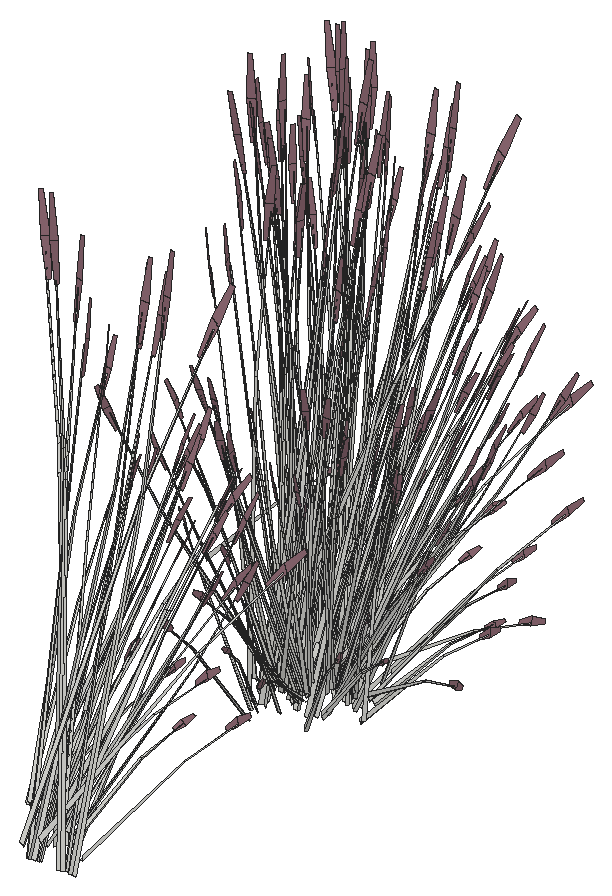
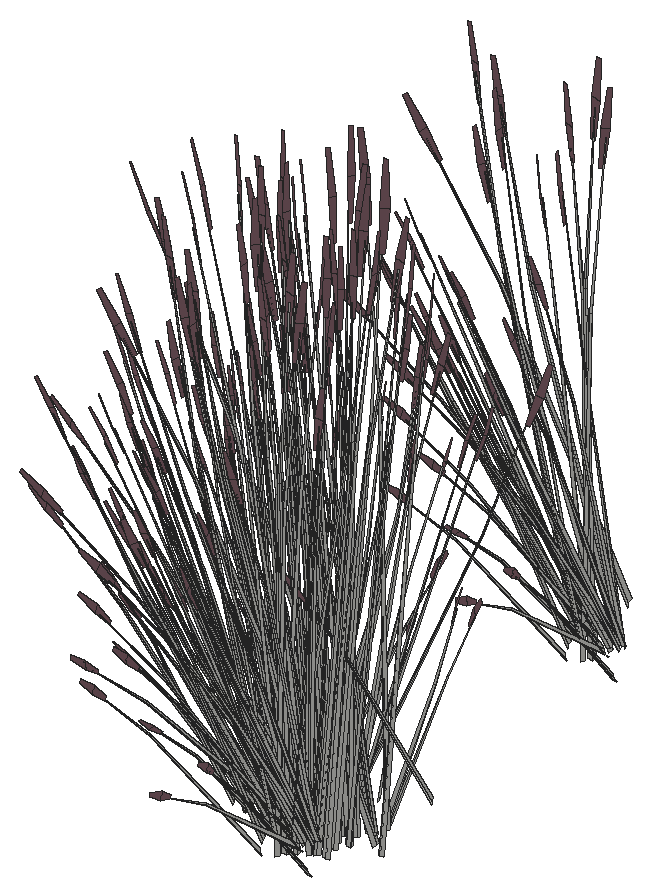
# SketchUp Ruby script. Lengths in inches.
U = 1.inch
M = Sketchup.active_model
def pt(a) = Geom::Point3d.new(a.map { |v| v * U })
def face(e, loops, mat)
  f = e.add_face(loops[0].map { |a| pt(a) })
  loops[1..].each { |l| e.add_face(l.map { |a| pt(a) }).erase! }
  f.material = f.back_material = mat if mat
  f
end
# faces: each face lists its corners as indices into pts; further lists are holes
def faces(e, pts, list, mat = nil) = list.each { |f| face(e, (f[0].is_a?(Array) ? f : [f]).map { |l| l.map { |i| pts[i] } }, mat) }
# xy, xz, yz: faces in a plane at the given z, y or x. An outline is a flat list of corners, or four numbers for a rectangle; further outlines are holes
def ring(l) = l.size == 4 ? [[l[0], l[1]], [l[2], l[1]], [l[2], l[3]], [l[0], l[3]]] : l.each_slice(2).to_a
def flat(e, list, mat, &to3) = list.each { |f| face(e, (f[0].is_a?(Array) ? f : [f]).map { |l| ring(l).map { |u, v| to3.(u, v) } }, mat) }
def xy(e, z, list, mat = nil) = flat(e, list, mat) { |x, y| [x, y, z] }
def xz(e, y, list, mat = nil) = flat(e, list, mat) { |x, z| [x, y, z] }
def yz(e, x, list, mat = nil) = flat(e, list, mat) { |y, z| [x, y, z] }
def lines(e, pts, list) = list.each { |a, b| e.add_line(pt(pts[a]), pt(pts[b])) }
# prism: a flat outline (further loops are holes) pulled along v
def prism(e, loops, v, mat = nil)
  f = face(e, loops, mat); d = Geom::Vector3d.new(v.map { |x| x * U })
  f.pushpull(f.normal.samedirection?(d) ? d.length : -d.length)
end
def box(e, o, s, mat = nil) = prism(e, [[o, [o[0] + s[0], o[1], o[2]], [o[0] + s[0], o[1] + s[1], o[2]], [o[0], o[1] + s[1], o[2]]]], [0, 0, s[2]], mat)
def at(x, y, z, deg = 0) = Geom::Transformation.translation(pt([x, y, z])) * Geom::Transformation.rotation(ORIGIN, Z_AXIS, deg.degrees)
def axes(o, x, y, z) = Geom::Transformation.new([*x, 0, *y, 0, *z, 0, *pt(o).to_a, 1])
def part(name) = M.definitions.add(name)
# library, detail: a bought-in or finely detailed component or shape, given as its bounding box
def library(name, o, s) = part(name).tap { |d| box(d.entities, o, s) }
def detail(e, o, s) = box(e.add_group.entities, o, s)
def put(e, d, t, mat = nil) = e.add_instance(d, t).tap { |i| i.material = mat if mat }
def group(e, t, mat = nil) = e.add_group.tap { |g| g.transformation = t; g.material = mat if mat }.entities
root = M.entities
M.materials.add("LightPink_Translucent").color = [144, 107, 117]
c1 = part("blade")
p = [[2.15,0.21,22],[0,0.17,0],[0.09,0.45,0],[2.18,0.31,22],[2.29,0.31,22],[0.38,0.45,0],
  [2.48,0.24,33],[2.49,0.24,33],[2.48,0.22,33]]
faces(c1.entities,p,[[0,1,2,3],[4,5,2,3],[6,3,4,7],[8,0,3,6]])
c2 = part("seeds")
p = [[0.3,-0.1,1.38],[-0.01,-0.03,1.59],[-0.01,-0.03,0.03],[0.14,-0.07,-0.07],[0.29,-0.03,3],[0.15,0.01,3.11]]
faces(c2.entities,p,[[0,1,2,3],[1,0,4,5]],"LightPink_Translucent")
c3 = part("blade with seeds")
put(c3.entities,c1,at(0,0,0))
put(c3.entities,c2,axes([2.4,0.25,30.99],[1.5799,-0.05474,1.17369],[-0.12525,1.92788,0.29478],[-0.07173,-0.02425,1.56792]))
put(root,c3,axes([64.18,687.89,43.49],[-0.06405,-0.15723,1.76342],[0.44421,-0.91974,-0.26939],[0.4481,-0.01323,0.30037]))
put(root,c3,axes([70.95,685.26,35.12],[0.85545,-0.64616,-0.30978],[0.85545,0.64616,0.30978],[0,-0.20813,1.38974]))
put(root,c3,axes([74.82,681.08,35.22],[-0.84686,0.59414,-0.03893],[-0.77596,-0.65071,-0.17649],[-0.05463,-0.18438,0.58215]))
put(root,c3,axes([74.48,686.94,35.45],[1.54892,0.2182,0.45755],[-0.31522,1.23236,0.17955],[-0.22636,-0.119,1.58856]))
put(root,c3,axes([74.08,686.72,35.81],[-0.59459,0.93321,0.44739],[-1.23546,-0.44912,-0.21531],[0,-0.21512,1.43643]))
put(root,c3,axes([76.04,682.22,38.07],[-0.5849,-0.8421,-0.71045],[1.20401,-0.4693,0.08574],[-0.13677,-0.40688,1.00501]))
put(root,c3,axes([73.65,688.91,35.56],[1.31687,-0.27488,0.17642],[0.32517,1.02297,0.35086],[-0.11745,-0.14905,1.60407]))
put(root,c3,axes([75.34,689.07,35.29],[-1.23546,-0.46496,0],[0.59459,-0.96613,0],[0,0,1.62707]))
put(root,c3,axes([76.27,682.34,38.14],[-0.36946,0.79643,0.35414],[-1.07787,-0.23229,-0.4572],[-0.09883,-0.32066,0.87481]))
put(root,c3,axes([78.2,650.68,36.17],[0.7662,1.03778,0],[-1.28187,0.57875,-0.51607],[-0.29196,0.13181,1.63711]))
put(root,c3,axes([78.2,690.24,35.46],[0.7662,1.03778,0],[-1.28187,0.57875,-0.51607],[-0.29196,0.13181,1.63711]))
put(root,c3,axes([74.3,651.13,38.86],[-1.20755,-0.27075,0.53283],[0.41292,-0.89013,0.43934],[0.07257,0.35005,1.10256]))
put(root,c3,axes([74.3,690.68,38.15],[-1.20755,-0.27075,0.53283],[0.41292,-0.89013,0.43934],[0.07257,0.35005,1.10256]))
put(root,c3,axes([73.98,651.2,38.52],[-0.90301,0.35198,0.0643],[-0.44199,-0.64184,0.50621],[0.08721,0.28293,0.77189]))
put(root,c3,axes([73.98,690.75,37.82],[-0.90301,0.35198,0.0643],[-0.44199,-0.64184,0.50621],[0.08721,0.28293,0.77189]))
put(root,c3,axes([77.5625,688.97,35.56],[0.35402,-1.02926,0.17642],[1.29548,0.29127,0.35086],[-0.22379,0.00501,1.60407]))
put(root,c3,axes([76.97,687.6,35.71],[0.90538,0.62224,0.1448],[-0.75521,0.70202,-0.41347],[-0.21021,0.09491,1.26744]))
put(root,c3,axes([76.64,686.83,35.39],[-1.1399,-0.8914,-0.06131],[1.1406,-0.89194,0],[-0.03981,-0.03113,1.75571]))
put(root,c3,axes([76.94,687.14,35.81],[1.33077,-0.06393,0.44739],[0.12035,1.06125,-0.21531],[-0.23824,0.10756,1.43643]))
put(root,c3,axes([77.27,650.03,36.125],[1.53422,0.33662,0.30756],[-0.38383,1.20322,-0.36492],[-0.25393,0.15059,1.64885]))
put(root,c3,axes([77.27,689.58,35.42],[1.53422,0.33662,0.30756],[-0.38383,1.20322,-0.36492],[-0.25393,0.15059,1.64885]))
put(root,c3,axes([75.03,680.35,34.58],[-0.20555,0.03731,1.76342],[-1.13672,-0.42002,-0.26939],[0.01907,-0.35034,0.30037]))
put(root,c3,axes([77.93,689.52,35.57],[1.14694,-0.51783,0.49651],[0.68554,0.92854,0],[-0.26122,0.11794,1.57504]))
put(root,c3,axes([76.15,681.51,37.62],[0.36946,-0.79643,-0.35414],[1.07787,0.23229,0.4572],[-0.09883,-0.32066,0.87481]))
put(root,c3,axes([74.34,685.81,35.45],[0.53281,1.15808,0.45755],[-1.52239,0.4027,0.17955],[0.01861,-0.2128,1.58856]))
put(root,c3,axes([74.1,685.66,35.3],[0.59459,-0.93321,-0.44739],[1.23546,0.44912,0.21531],[0,-0.21512,1.43643]))
put(root,c3,axes([75.62,688.67,35.29],[-0.39985,-0.89288,0],[1.1418,-0.31268,0],[0,0,1.54371]))
put(root,c3,axes([74.17,651,35.29],[0.19833,-0.05635,1.76342],[1.19302,0.31018,-0.26939],[0.03489,0.3496,0.30037]))
put(root,c3,axes([74.17,690.55,34.58],[0.19833,-0.05635,1.76342],[1.19302,0.31018,-0.26939],[0.03489,0.3496,0.30037]))
put(root,c3,axes([74.43,651.3125,38.32],[-0.36946,0.79643,-0.35414],[-1.07787,-0.23229,0.4572],[0.09883,0.32066,0.87481]))
put(root,c3,axes([74.43,690.87,37.62],[-0.36946,0.79643,-0.35414],[-1.07787,-0.23229,0.4572],[0.09883,0.32066,0.87481]))
put(root,c3,axes([77.24,647.35,36],[-0.59459,0.93321,-0.44739],[-1.23546,-0.44912,0.21531],[0,0.21512,1.43643]))
put(root,c3,axes([77.24,686.91,35.3],[-0.59459,0.93321,-0.44739],[-1.23546,-0.44912,0.21531],[0,0.21512,1.43643]))
put(root,c3,axes([76.6,681.62,37.82],[0.90301,-0.35198,0.0643],[0.44199,0.64184,0.50621],[-0.08721,-0.28293,0.77189]))
put(root,c3,axes([73.67,652.72,38.51],[0.15534,0.16677,1.74944],[1.25362,0.06552,-0.27667],[0.12606,0.3678,0.14031]))
put(root,c3,axes([73.67,692.28,37.81],[0.15534,0.16677,1.74944],[1.25362,0.06552,-0.27667],[0.12606,0.3678,0.14031]))
put(root,c3,axes([79.59,686.34,35.56],[-0.96285,-0.75439,0.17642],[0.97031,-0.7317,0.35086],[-0.10634,0.15406,1.60407]))
put(root,c3,axes([76.26,685.9,35.3],[0,-1.19833,0],[1.53239,0,0],[0,0,1.79456]))
put(root,c3,axes([76.28,681.69,37.82],[1.20755,0.27075,0.48003],[-0.41292,0.89013,0.3958],[-0.07257,-0.35005,0.9933]))
put(root,c3,axes([74.84,686.12,35.52],[1.3808,0.50196,0.24065],[-0.66454,1.04299,0.50002],[0,-0.24043,1.60543]))
put(root,c3,axes([77.03,686.38,35.38],[0,1.19774,-0.05637],[-1.53239,0,0],[0,0.03764,1.79368]))
put(root,c3,axes([74.39,685.42,35.81],[-1.33077,0.06393,0.44739],[-0.12035,-1.06125,-0.21531],[0.23824,-0.10756,1.43643]))
put(root,c3,axes([74.3125,650.47,38.84],[0.36946,-0.79643,0.35414],[1.07787,0.23229,-0.4572],[0.09883,0.32066,0.87481]))
put(root,c3,axes([74.3125,690.03,38.14],[0.36946,-0.79643,0.35414],[1.07787,0.23229,-0.4572],[0.09883,0.32066,0.87481]))
put(root,c3,axes([73.77,683.6,35.56],[-0.35402,1.02926,0.17642],[-1.29548,-0.29127,0.35086],[0.22379,-0.00501,1.60407]))
put(root,c3,axes([76.3,688.7,35.38],[0.53281,1.18979,-0.06012],[-1.52239,0.41691,0],[0.01861,0.04155,1.72173]))
put(root,c3,axes([73.14,682.33,35.46],[-0.7662,-1.03778,0],[1.28187,-0.57875,-0.51607],[0.29196,-0.13181,1.63711]))
put(root,c3,axes([74.54,650.6,38.77],[0.5849,0.8421,-0.71045],[-1.20401,0.4693,0.08574],[0.13677,0.40688,1.00501]))
put(root,c3,axes([74.54,690.15,38.07],[0.5849,0.8421,-0.71045],[-1.20401,0.4693,0.08574],[0.13677,0.40688,1.00501]))
put(root,c3,axes([80.7,647.58,35.99],[-1.53164,-0.00828,-0.04976],[0,-1.1575,0.49943],[-0.04813,0.2635,1.58352]))
put(root,c3,axes([80.7,687.14,35.29],[-1.53164,-0.00828,-0.04976],[0,-1.1575,0.49943],[-0.04813,0.2635,1.58352]))
put(root,c3,axes([77.6875,683.66,35.56],[-1.31687,0.27488,0.17642],[-0.32517,-1.02297,0.35086],[0.11745,0.14905,1.60407]))
put(root,c3,axes([76.34,679.82,35.86],[0.15721,0.60392,1.1486],[-0.87211,-0.33448,0.84392],[0.09385,-0.30923,0.25299]))
put(root,c3,axes([75.76,653.31,39.44],[0.84686,-0.59414,-0.06488],[0.77596,0.65071,-0.29416],[0.05463,0.18438,0.97024]))
put(root,c3,axes([75.76,692.87,38.74],[0.84686,-0.59414,-0.06488],[0.77596,0.65071,-0.29416],[0.05463,0.18438,0.97024]))
put(root,c3,axes([75.53,685.15,35.45],[-1.01611,0.93987,0.45755],[-1.20717,-0.82966,0.17955],[0.24496,-0.0938,1.58856]))
put(root,c3,axes([77.27,686.63,35.31],[0.85545,0.66896,0],[-0.85545,0.66896,0],[0,0,1.69266]))
put(root,c3,axes([77.26,685.85,35.81],[0.59459,-0.93321,0.44739],[1.23546,0.44912,-0.21531],[0,0.21512,1.43643]))
put(root,c3,axes([76.74,689.09,35.29],[1.23546,0.46496,0],[-0.59459,0.96613,0],[0,0,1.74954]))
put(root,c3,axes([74.98,650.77,38.47],[1.20468,0.25962,-0.51099],[-0.41292,0.89013,-0.3958],[0.11046,0.35838,0.97773]))
put(root,c3,axes([74.98,690.32,37.77],[1.20468,0.25962,-0.51099],[-0.41292,0.89013,-0.3958],[0.11046,0.35838,0.97773]))
put(root,c3,axes([73.95,650.81,38.83],[1.19922,-0.48218,-0.1216],[0.58932,0.85579,-0.67495],[0.15822,0.36063,1.02557]))
put(root,c3,axes([73.95,690.36,38.125],[1.19922,-0.48218,-0.1216],[0.58932,0.85579,-0.67495],[0.15822,0.36063,1.02557]))
put(root,c3,axes([76.86,685.625,35.47],[-1.54892,-0.2182,0.49198],[0.31522,-1.23236,0.19306],[0.22636,0.119,1.70813]))
put(root,c3,axes([80.08,680.81,37.8],[-0.12446,0.07911,1.77383],[-1.21937,-0.26689,-0.16761],[-0.04414,-0.34521,0.31391]))
put(root,c3,axes([79.12,683.09,38.125],[-1.34686,-0.05131,-0.1216],[0.03681,-0.97156,-0.67495],[0.09356,-0.37418,1.02557]))
put(root,c3,axes([80.38,647.75,35.82],[-0.85545,0.64616,-0.30978],[-0.85545,-0.64616,0.30978],[0,0.20813,1.38974]))
put(root,c3,axes([80.38,687.31,35.12],[-0.85545,0.64616,-0.30978],[-0.85545,-0.64616,0.30978],[0,0.20813,1.38974]))
put(root,c3,axes([77.94,647.63,35.89],[0.44936,0.94823,-0.69212],[-1.29441,0.3415,-0.18165],[0.04967,0.32109,1.52773]))
put(root,c3,axes([77.94,687.1875,35.19],[0.44936,0.94823,-0.69212],[-1.29441,0.3415,-0.18165],[0.04967,0.32109,1.52773]))
put(root,c3,axes([77.3,686.17,35.3],[1.37109,0,0],[0,1.07219,0],[0,0,1.78407]))
put(root,c3,axes([78.59,683.24,38.14],[-0.82919,0.54528,0.35414],[-0.78493,-0.62262,-0.4572],[0.11943,-0.31634,0.87481]))
put(root,c3,axes([75.98,684.99,35.81],[-0.73619,-0.86927,0.44739],[1.11511,-0.61213,-0.21531],[0.23824,0.10756,1.43643]))
put(root,c3,axes([74.64,685.2,35.76],[-0.1428,-1.18174,-0.29095],[1.48733,-0.07145,-0.50002],[0.26191,-0.15741,1.59708]))
put(root,c3,axes([77.77,686.0625,35.71],[1.1418,-0.30203,0.1448],[0.39985,0.86246,-0.41347],[0,0.18981,1.26744]))
put(root,c3,axes([78.2,682.73,37.77],[-0.87728,-0.69587,-0.51099],[0.92674,-0.60943,-0.3958],[0.13348,-0.35356,0.97773]))
put(root,c3,axes([77.38,646.58,36.46],[1.38012,0.49416,-0.29095],[-0.66454,1.04299,-0.50002],[0.04337,0.25608,1.59708]))
put(root,c3,axes([77.38,686.13,35.76],[1.38012,0.49416,-0.29095],[-0.66454,1.04299,-0.50002],[0.04337,0.25608,1.59708]))
put(root,c3,axes([74.45,682.58,35.12],[1.14332,0.25625,-0.30978],[-0.28787,0.90242,0.30978],[0.23049,-0.10406,1.38974]))
put(root,c3,axes([77.625,681.49,35.68],[-0.34835,0.20963,1.43002],[-1.04325,-0.36691,-0.30754],[0.19338,-0.4563,0.61141]))
put(root,c3,axes([80.38,686.37,35.57],[0,-1.03566,0.49651],[1.37109,0,0],[0,0.23588,1.57504]))
put(root,c3,axes([80.97,647.78,35.8125],[0,1.03566,-0.49651],[-1.37109,0,0],[0,0.23588,1.57504]))
put(root,c3,axes([80.97,687.33,35.11],[0,1.03566,-0.49651],[-1.37109,0,0],[0,0.23588,1.57504]))
put(root,c3,axes([77.31,650.91,38.53],[-1.21888,0.23767,0.48003],[-0.21154,-0.93233,0.3958],[0.28666,0.27478,0.9933]))
put(root,c3,axes([77.31,690.47,37.82],[-1.21888,0.23767,0.48003],[-0.21154,-0.93233,0.3958],[0.28666,0.27478,0.9933]))
put(root,c3,axes([74.18,682.17,35.11],[1.14694,-0.51783,-0.49651],[0.68554,0.92854,0],[0.26122,-0.11794,1.57504]))
put(root,c3,axes([77.07,651.1,38.52],[-0.55698,0.6579,0.0643],[-0.79316,-0.38303,0.50621],[0.25643,0.21093,0.77189]))
put(root,c3,axes([77.07,690.65,37.82],[-0.55698,0.6579,0.0643],[-0.79316,-0.38303,0.50621],[0.25643,0.21093,0.77189]))
put(root,c3,axes([75.66,648.93,37.67],[-0.28013,-0.33252,1.71376],[1.29445,-0.27994,0.13857],[0.29256,0.52202,0.73262]))
put(root,c3,axes([75.66,688.48,36.97],[-0.28013,-0.33252,1.71376],[1.29445,-0.27994,0.13857],[0.29256,0.52202,0.73262]))
put(root,c3,axes([76.48,684.74,35.71],[0.23642,-0.92427,0.1448],[1.15506,0.16044,-0.41347],[0.21021,0.09491,1.26744]))
put(root,c3,axes([78.12,683.13,35.57],[-1.14694,-0.51783,0.49651],[0.68554,-0.92854,0],[0.26122,0.11794,1.57504]))
put(root,c3,axes([78.47,683.04,38.07],[0.03189,-0.95798,-0.71045],[1.34277,0.06434,0.08574],[0.14171,-0.40585,1.00501]))
put(root,c3,axes([77.12,688.54,35.28],[1.2866,-0.3514,-0.19198],[0.45209,1.01223,0.00008],[0.14202,-0.03884,1.73897]))
put(root,c3,axes([76.9,650.34,38.84],[-0.18927,-0.83419,0.35414],[1.08199,-0.22027,-0.4572],[0.29062,0.23905,0.87481]))
put(root,c3,axes([76.9,689.9,38.14],[-0.18927,-0.83419,0.35414],[1.08199,-0.22027,-0.4572],[0.29062,0.23905,0.87481]))
put(root,c3,axes([77.14,685.53,35.3],[0.73619,0.86927,-0.44739],[-1.11511,0.61213,0.21531],[0.23824,0.10756,1.43643]))
put(root,c3,axes([77.63,645.54,38.27],[-1.05895,-0.53811,1.38283],[1.11816,-0.83781,0.59665],[0.34166,0.5049,1.33663]))
put(root,c3,axes([77.63,685.1,37.5625],[-1.05895,-0.53811,1.38283],[1.11816,-0.83781,0.59665],[0.34166,0.5049,1.33663]))
put(root,c3,axes([79.03,682.47,37.62],[0.82919,-0.54528,-0.35414],[0.78493,0.62262,0.4572],[0.11943,-0.31634,0.87481]))
put(root,c3,axes([75.85,651.51,38.5],[0.00363,-0.12539,1.77383],[1.0502,-0.55319,-0.16761],[0.36479,0.19745,0.31391]))
put(root,c3,axes([75.85,691.0625,37.8],[0.00363,-0.12539,1.77383],[1.0502,-0.55319,-0.16761],[0.36479,0.19745,0.31391]))
put(root,c3,axes([79.35,682.75,37.82],[1.00708,0.04826,0.0643],[-0.02761,0.72867,0.50621],[0.10538,-0.27912,0.77189]))
put(root,c3,axes([79.23,649.92,36.56],[-0.69001,-0.29779,1.1486],[0.89096,-0.30257,0.84392],[0.24031,0.2563,0.25299]))
put(root,c3,axes([79.23,689.48,35.86],[-0.69001,-0.29779,1.1486],[0.89096,-0.30257,0.84392],[0.24031,0.2563,0.25299]))
put(root,c3,axes([76.77,649.61,36.38],[0.02163,-0.34331,1.43002],[1.03345,-0.38348,-0.30754],[0.31903,0.4109,0.61141]))
put(root,c3,axes([76.77,689.16,35.68],[0.02163,-0.34331,1.43002],[1.03345,-0.38348,-0.30754],[0.31903,0.4109,0.61141]))
put(root,c3,axes([80.35,681.55,37.81],[-0.01183,-0.20612,1.74944],[-0.99913,-0.59572,-0.27667],[0.15447,-0.36112,0.14031]))
put(root,c3,axes([75.54,684.29,35.15],[0.82544,-0.77843,-0.62353],[1.0254,0.70586,-0.16365],[0.33076,-0.19418,1.37633]))
put(root,c3,axes([79.02,682.68,37.82],[0.87265,0.70663,0.48003],[-0.92674,0.60943,0.3958],[0.16097,-0.33153,0.9933]))
put(root,c3,axes([79.16,683.6,35.12],[0.28787,0.90242,-0.30978],[-1.14332,0.25625,0.30978],[0.23049,0.10406,1.38974]))
put(root,c3,axes([81.31,646.99,36.17],[1.53239,0,0],[0,1.1575,-0.51607],[0,0.26363,1.63711]))
put(root,c3,axes([81.31,686.54,35.47],[1.53239,0,0],[0,1.1575,-0.51607],[0,0.26363,1.63711]))
put(root,c3,axes([76.36,685.04,35.76],[1.23732,-0.68758,-0.29095],[0.8228,0.97154,-0.50002],[0.30528,0.09867,1.59708]))
put(root,c3,axes([79.34,651.28,36.46],[-0.78586,-0.03248,1.0506],[0.51898,-0.68985,0.58006],[0.31045,0.24509,0.8241]))
put(root,c3,axes([79.34,690.83,35.76],[-0.78586,-0.03248,1.0506],[0.51898,-0.68985,0.58006],[0.31045,0.24509,0.8241]))
put(root,c3,axes([80.03,684.93,38.14],[-1.06674,0.14801,0.35414],[-0.28168,-0.84611,-0.4572],[0.30569,-0.22726,0.87481]))
put(root,c3,axes([76.96,682.56,36.97],[-0.22818,0.35597,1.71376],[-0.95725,-0.73667,0.13857],[0.43183,-0.45914,0.73262]))
put(root,c3,axes([76.8,650.77,38.83],[0.73026,-0.88648,-0.1216],[1.05755,0.51071,-0.67495],[0.36761,0.25045,1.02557]))
put(root,c3,axes([76.8,690.33,38.125],[0.73026,-0.88648,-0.1216],[1.05755,0.51071,-0.67495],[0.36761,0.25045,1.02557]))
put(root,c3,axes([73.23,684.43,34.68],[-1.20625,0.41464,1.28929],[-0.38394,-1.1897,0.50096],[0.74071,0.01979,1.46642]))
put(root,c3,axes([80.59,685,38.125],[-1.1336,-0.57106,-0.1216],[0.65308,-0.827,-0.67495],[0.32027,-0.28747,1.02557]))
put(root,c3,axes([77.67,650.33,38.47],[1.20928,-0.24619,-0.51099],[0.21154,0.93233,-0.3958],[0.32481,0.26718,0.97773]))
put(root,c3,axes([77.67,689.89,37.77],[1.20928,-0.24619,-0.51099],[0.21154,0.93233,-0.3958],[0.32481,0.26718,0.97773]))
put(root,c3,axes([78.78,682.59,35.47],[0.7662,-1.03778,0],[1.28187,0.57875,-0.51607],[0.29196,0.13181,1.63711]))
put(root,c3,axes([80.0625,682.14,34.58],[-0.18342,-0.08159,1.76342],[-0.47115,-0.9115,-0.26939],[0.31784,-0.24736,0.30037]))
put(root,c3,axes([79.06,688.77,38.14],[-0.69728,-0.64842,0.35414],[0.79619,-0.61382,-0.4572],[0.40453,0.09339,0.87481]))
put(root,c3,axes([79.48,683.22,35.11],[1.14694,0.51783,-0.49651],[-0.68554,0.92854,0],[0.26122,0.11794,1.57504]))
put(root,c3,axes([79.6875,649.8,38.52],[-0.06171,0.78753,0.0643],[-0.9318,-0.02159,0.50621],[0.35694,0.08241,0.77189]))
put(root,c3,axes([79.6875,689.36,37.82],[-0.06171,0.78753,0.0643],[-0.9318,-0.02159,0.50621],[0.35694,0.08241,0.77189]))
put(root,c3,axes([79.42,651.03,35.29],[0.08928,-0.14952,1.76342],[1.12407,-0.44035,-0.26939],[0.34078,0.22791,0.30037]))
put(root,c3,axes([79.42,690.58,34.58],[0.08928,-0.14952,1.76342],[1.12407,-0.44035,-0.26939],[0.34078,0.22791,0.30037]))
put(root,c3,axes([79.77,649.55,38.53],[-0.90362,0.68241,0.48003],[-0.77932,-0.72471,0.3958],[0.42395,0.12588,0.9933]))
put(root,c3,axes([79.77,689.11,37.82],[-0.90362,0.68241,0.48003],[-0.77932,-0.72471,0.3958],[0.42395,0.12588,0.9933]))
put(root,c3,axes([80.02,684.33,37.77],[-0.31482,-0.94565,-0.51099],[1.19224,-0.16542,-0.3958],[0.34166,-0.254,0.97773]))
put(root,c3,axes([82.12,689.21,37.02],[-0.23455,-0.87059,-0.03492],[1.10861,-0.20015,-0.15832],[0.23151,0.05519,0.52218]))
put(root,c3,axes([80.2,686.95,38.14],[-1.01846,-0.28891,0.35414],[0.29705,-0.84289,-0.4572],[0.41005,-0.07729,0.87481]))
put(root,c3,axes([77.8,685.2,35.15],[1.27479,0.1698,-0.62353],[-0.26901,1.04736,-0.16365],[0.38043,0.12691,1.37633]))
put(root,c3,axes([83.23,685.82,35.35],[-0.75977,-0.66224,-0.06488],[0.83212,-0.6068,-0.29416],[0.23578,-0.04272,0.97024]))
put(root,c3,axes([81.49,682.45,35.86],[-0.40819,0.5272,1.1486],[-0.35086,-0.70831,0.84392],[0.33713,-0.17749,0.25299]))
put(root,c3,axes([81,684.79,37.82],[0.8413,0.43556,0.0643],[-0.48981,0.62025,0.50621],[0.26973,-0.20053,0.77189]))
put(root,c3,axes([80.77,684.61,37.82],[0.30393,0.95317,0.48003],[-1.19224,0.16542,0.3958],[0.35138,-0.22417,0.9933]))
put(root,c3,axes([77.54,647.89,37.67],[-0.45521,-0.17844,1.71376],[0.94204,-0.74856,0.13857],[0.58713,0.33769,0.73262]))
put(root,c3,axes([77.54,687.45,36.97],[-0.45521,-0.17844,1.71376],[0.94204,-0.74856,0.13857],[0.58713,0.33769,0.73262]))
put(root,c3,axes([83.38,684.76,37.8],[-0.16006,-0.00787,1.77383],[-0.66468,-0.8428,-0.16761],[0.26693,-0.27711,0.31391]))
put(root,c3,axes([80.9,684.43,37.62],[1.06674,-0.14801,-0.35414],[0.28168,0.84611,0.4572],[0.30569,-0.22726,0.87481]))
put(root,c3,axes([80.06,684.71,38.07],[0.64013,-0.81717,-0.71045],[1.12174,0.58074,0.08574],[0.38221,-0.29607,1.00501]))
put(root,c3,axes([81.125,687.21,37.82],[0.4501,0.70615,0.0643],[-0.82077,0.34564,0.50621],[0.36181,-0.0682,0.77189]))
put(root,c3,axes([80.05,649.55,38.32],[0.69728,0.64842,-0.35414],[-0.79619,0.61382,0.4572],[0.40453,0.09339,0.87481]))
put(root,c3,axes([80.05,689.11,37.62],[0.69728,0.64842,-0.35414],[-0.79619,0.61382,0.4572],[0.40453,0.09339,0.87481]))
put(root,c3,axes([79.25,689.18,38.125],[0.06562,-1.05324,-0.1216],[1.2424,0.02879,-0.67495],[0.4785,0.07316,1.02557]))
put(root,c3,axes([80.63,687.23,38.125],[-0.6166,-0.93779,-0.1216],[1.09436,-0.46085,-0.67495],[0.46117,-0.12373,1.02557]))
put(root,c3,axes([81.04,686.96,37.82],[-0.34623,0.9443,0.48003],[-1.13828,-0.3229,0.3958],[0.44763,-0.05675,0.9933]))
put(root,c3,axes([80.33,688.55,37.81],[0.26289,-0.01751,1.74944],[0.72108,-0.8046,-0.27667],[0.46761,0.10621,0.14031]))
put(root,c3,axes([80.58,686.43,37.77],[0.332,-0.94205,-0.51099],[1.13828,0.3229,-0.3958],[0.45829,-0.08638,0.97773]))
put(root,c3,axes([83.4375,687.03,35.86],[-0.75718,0.17097,1.1486],[0.35641,-0.70661,0.84392],[0.40168,0.04835,0.25299]))
put(root,c3,axes([80.98,683.96,35.68],[-0.4378,-0.03068,1.43002],[-0.44851,-0.8229,-0.30754],[0.53783,-0.23279,0.61141]))
put(root,c3,axes([81.28,686.86,37.62],[1.01846,0.28891,-0.35414],[-0.29705,0.84289,0.4572],[0.41005,-0.07729,0.87481]))
put(root,c3,axes([79.31,688.68,38.07],[1.22504,0.02494,-0.71045],[-0.08228,1.05005,0.08574],[0.51899,0.11081,1.00501]))
put(root,c3,axes([81.79,686.69,35.07],[-0.7893,0.12429,1.41583],[-0.12563,-0.9893,0.08104],[0.55282,-0.14974,0.80566]))
put(root,c3,axes([82.66,686.05,34.58],[-0.06405,-0.15723,1.76342],[0.44421,-0.91974,-0.26939],[0.4481,-0.01323,0.30037]))
put(root,c3,axes([83.08,690.02,37.8],[-0.11081,-0.09067,1.77383],[0.2424,-0.97188,-0.16761],[0.43649,-0.06209,0.31391]))
put(root,c3,axes([78.5,685.8125,36.97],[-0.50831,0.02346,1.71376],[0.33721,-1.01661,0.13857],[0.72439,0.06288,0.73262]))
put(root,c3,axes([80.36,686.77,38.07],[1.07686,-0.45739,-0.71045],[0.60013,0.94154,0.08574],[0.52031,-0.10696,1.00501]))
put(root,c3,axes([83.98,685.76,37.81],[0.17006,-0.15775,1.74944],[-0.21766,-0.96766,-0.27667],[0.42669,-0.18347,0.14031]))
put(root,c3,axes([82.02,688.16,35.68],[-0.29514,-0.25472,1.43002],[0.38401,-0.84262,-0.30754],[0.59714,0.11414,0.61141]))
